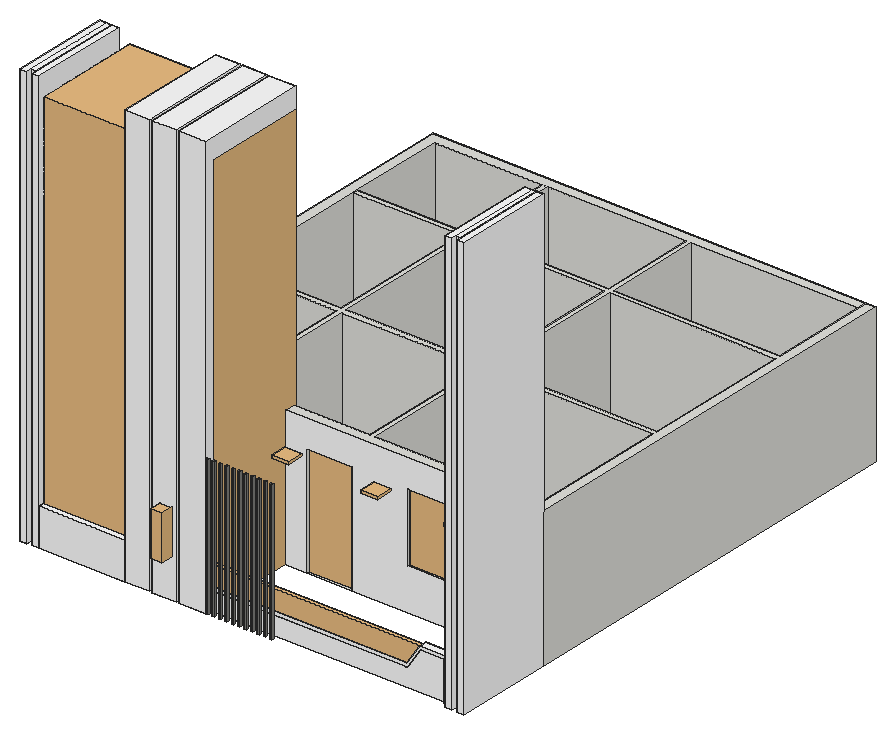
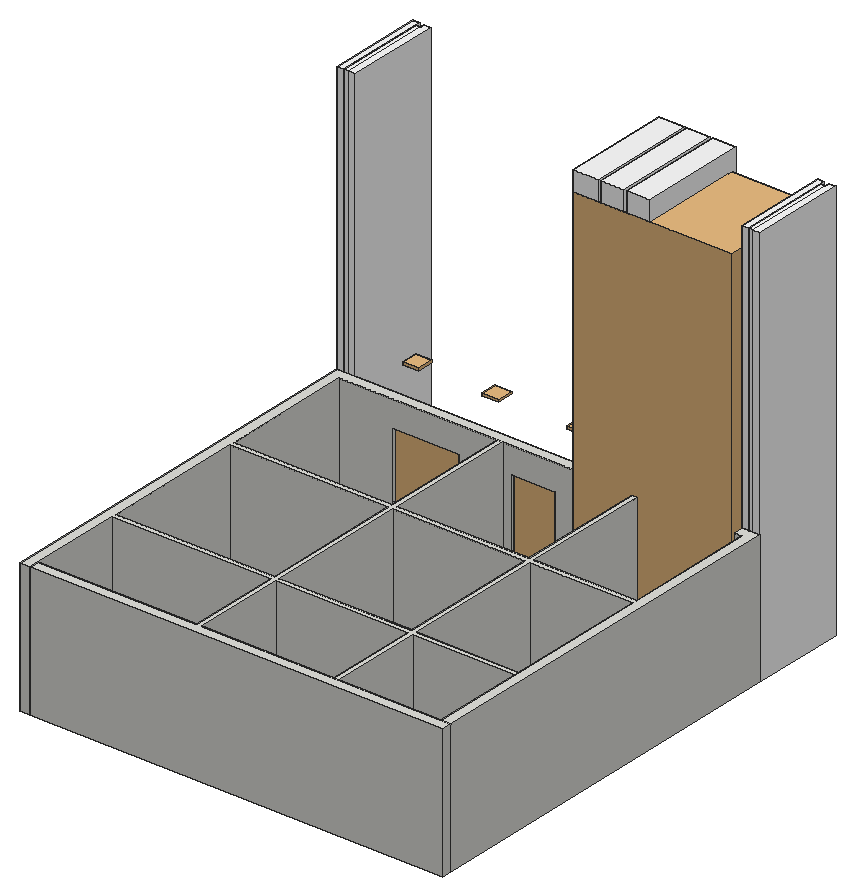
# SketchUp Ruby script. Lengths in inches.
U = 1.inch
M = Sketchup.active_model
def pt(a) = Geom::Point3d.new(a.map { |v| v * U })
def face(e, loops, mat)
  f = e.add_face(loops[0].map { |a| pt(a) })
  loops[1..].each { |l| e.add_face(l.map { |a| pt(a) }).erase! }
  f.material = f.back_material = mat if mat
  f
end
# faces: each face lists its corners as indices into pts; further lists are holes
def faces(e, pts, list, mat = nil) = list.each { |f| face(e, (f[0].is_a?(Array) ? f : [f]).map { |l| l.map { |i| pts[i] } }, mat) }
# xy, xz, yz: faces in a plane at the given z, y or x. An outline is a flat list of corners, or four numbers for a rectangle; further outlines are holes
def ring(l) = l.size == 4 ? [[l[0], l[1]], [l[2], l[1]], [l[2], l[3]], [l[0], l[3]]] : l.each_slice(2).to_a
def flat(e, list, mat, &to3) = list.each { |f| face(e, (f[0].is_a?(Array) ? f : [f]).map { |l| ring(l).map { |u, v| to3.(u, v) } }, mat) }
def xy(e, z, list, mat = nil) = flat(e, list, mat) { |x, y| [x, y, z] }
def xz(e, y, list, mat = nil) = flat(e, list, mat) { |x, z| [x, y, z] }
def yz(e, x, list, mat = nil) = flat(e, list, mat) { |y, z| [x, y, z] }
def lines(e, pts, list) = list.each { |a, b| e.add_line(pt(pts[a]), pt(pts[b])) }
# prism: a flat outline (further loops are holes) pulled along v
def prism(e, loops, v, mat = nil)
  f = face(e, loops, mat); d = Geom::Vector3d.new(v.map { |x| x * U })
  f.pushpull(f.normal.samedirection?(d) ? d.length : -d.length)
end
def box(e, o, s, mat = nil) = prism(e, [[o, [o[0] + s[0], o[1], o[2]], [o[0] + s[0], o[1] + s[1], o[2]], [o[0], o[1] + s[1], o[2]]]], [0, 0, s[2]], mat)
def at(x, y, z, deg = 0) = Geom::Transformation.translation(pt([x, y, z])) * Geom::Transformation.rotation(ORIGIN, Z_AXIS, deg.degrees)
def axes(o, x, y, z) = Geom::Transformation.new([*x, 0, *y, 0, *z, 0, *pt(o).to_a, 1])
def part(name) = M.definitions.add(name)
# library, detail: a bought-in or finely detailed component or shape, given as its bounding box
def library(name, o, s) = part(name).tap { |d| box(d.entities, o, s) }
def detail(e, o, s) = box(e.add_group.entities, o, s)
def put(e, d, t, mat = nil) = e.add_instance(d, t).tap { |i| i.material = mat if mat }
def group(e, t, mat = nil) = e.add_group.tap { |g| g.transformation = t; g.material = mat if mat }.entities
root = M.entities
M.materials.add("Ecorel - epc61025 33.57cm").color = [255, 255, 255]
M.materials.add("Foil Dark Green Matte 0.01cm").color = [255, 255, 255]
M.materials.add("Iron Rough 15cm").color = [129, 129, 125]
M.materials.add("Kamosho - kamn7918 33.43cm").color = [255, 255, 255]
M.materials.add("Leather Brown Alcantara 003 9.18cm").color = [255, 255, 255]
M.materials.add("Pp-1846-msg 17.72cm").color = [255, 255, 255]
c1 = library("Window Crafter Sliding",[0,-0.55,0],[60,4.49,60])
c2 = library("Door 243 065",[-19.36,-2.49,0],[38.72,4.98,81.96])
c3 = library("Group\#13",[0,4.3125,0],[144.25,93,348])
c4 = part("Group\#15")
prism(c4.entities,[[[-3.75,7.71,0],[-3.75,0,0],[-3.75,0,365.875],[-3.75,97.71,365.875],[-3.75,97.71,348],[-3.75,7.71,348]]],[21.11,0,0])
c5 = part("Vertical post")
box(c5.entities,[0,0.5,0],[2,1.5,120],"Iron Rough 15cm")
c6 = part("Stair tread")
box(c6.entities,[0,0,0],[12,36,7])
c7 = part("Stair tread \#1")
box(c7.entities,[0,0,0],[19.0625,36,7])
c8 = part("Stair landing")
box(c8.entities,[-12.25,0,0],[24.25,74,7])
c9 = library("Group\#40",[0,0,0],[184.84,3.15,25.98])
c10 = library("Group\#44",[0,0,0],[10.21,10.4,38.37])
c11 = library("Tlon Light 650 Ceiling 152 007",[-12.8,-12.8,-3.78],[25.6,25.6,3.58])
xy(root,132,[[689.2,386.76,763.65,394.47],[1035.98,391.51,1035.98,391.76,833.45,391.76,833.45,398.76,1040.7,398.76,1040.7,391.51]])
xy(root,148.48,[[833.45,391.51,1004.61,391.76]])
xy(root,151,[[833.45,391.51,1003.26,398.76]],"Foil Dark Green Matte 0.01cm")
xy(root,164.8125,[[689.2,386.76,763.65,394.47]],"Leather Brown Alcantara 003 9.18cm")
xy(root,165.48,[[1015.86,391.51,1035.98,391.76]])
xy(root,168,[[1014.5,391.51,1040.7,398.76]],"Foil Dark Green Matte 0.01cm")
xz(root,386.76,[[689.2,132,763.65,164.8125]],"Leather Brown Alcantara 003 9.18cm")
xz(root,391.51,[[1035.98,132,1040.7,132,1040.7,168,1014.5,168,1003.26,151,833.45,151,833.45,148.48,1004.61,148.48,1015.86,165.48,1035.98,165.48]],"Foil Dark Green Matte 0.01cm")
xz(root,391.76,[[833.45,132,1035.98,132,1035.98,165.48,1015.86,165.48,1004.61,148.48,833.45,148.48]],"Kamosho - kamn7918 33.43cm")
xz(root,394.47,[[689.2,132,763.65,164.8125]])
xz(root,398.76,[[833.45,132,833.45,151,1003.26,151,1014.5,168,1040.7,168,1040.7,132]])
yz(root,689.2,[[386.76,132,394.47,164.8125]])
yz(root,763.65,[[386.76,132,394.47,164.8125]])
yz(root,833.45,[[391.76,132,391.76,148.48,391.51,148.48,391.51,151,398.76,151,398.76,132]])
yz(root,1035.98,[[391.51,132,391.76,165.48]])
yz(root,1040.7,[[391.51,132,398.76,168]])
p = [[1004.61,391.76,148.48],[1015.86,391.76,165.48],[1015.86,391.51,165.48],[1004.61,391.51,148.48],[1003.26,398.76,151],[1003.26,391.51,151],
  [1014.5,391.51,168],[1014.5,398.76,168]]
faces(root,p,[[0,1,2,3]])
faces(root,p,[[4,5,6,7]],"Foil Dark Green Matte 0.01cm")
g1 = group(root,at(672.95,472.76,132))
put(g1,c1,at(266.5625,2.73,36))
put(g1,c2,axes([198.48,4.93,0],[1,0,0],[0,1,0],[0,0,1.17128]))
g2 = group(g1,at(0,0,0))
xy(g2,0,[[179.1875,0,218.1875,9],[9,9,102,129],[106.5,9,226.5,129],[231,9,375,129],[9,133.5,102,262.5],
  [106.5,133.5,226.5,262.5],[231,133.5,375,262.5],[9,267,102,351],[106.5,267,226.5,351],[231,267,375,351]])
xy(g2,36,[[266.5625,0,326.5625,9]])
xy(g2,96,[[179.1875,0,218.1875,9],[266.5625,0,326.5625,9]])
xy(g2,120,[[[0,0,384,0,384,360,375,360,375,267,231,267,231,351,375,351,375,360,0,360,0,351,226.5,351,226.5,267,106.5,267,106.5,351,102,351,102,267,9,267,9,262.5,102,262.5,102,133.5,9,133.5,9,351,0,351],[106.5,9,106.5,129,226.5,129,226.5,9,231,9,231,129,375,129,375,9],[231,133.5,375,262.5],[106.5,133.5,226.5,262.5],[9,9,102,129]]])
xz(g2,0,[[[0,0,179.1875,0,179.1875,96,218.1875,96,218.1875,0,384,0,384,120,0,120],[266.5625,36,326.5625,96]]],"Pp-1846-msg 17.72cm")
xz(g2,9,[[9,0,102,120],[106.5,0,106.5,120,226.5,120,226.5,0,218.1875,0,218.1875,96,179.1875,96,179.1875,0],[226.5,0,231,120],[[231,0,375,120],[266.5625,36,326.5625,96]]])
xz(g2,129,[[9,0,102,120],[106.5,0,226.5,120],[231,0,375,120]])
xz(g2,133.5,[[9,0,102,120],[106.5,0,226.5,120],[231,0,375,120]])
xz(g2,262.5,[[9,0,102,120],[106.5,0,226.5,120],[231,0,375,120]])
xz(g2,267,[[9,0,102,120],[106.5,0,226.5,120],[231,0,375,120]])
xz(g2,351,[[0,0,9,120],[9,0,102,120],[102,0,106.5,120],[106.5,0,226.5,120],[231,0,375,120]])
xz(g2,360,[[0,0,375,120],[375,0,384,120]])
yz(g2,0,[[0,0,351,120],[351,0,360,120]])
yz(g2,9,[[9,0,129,120],[133.5,0,262.5,120],[262.5,0,267,120],[267,0,351,120]])
yz(g2,102,[[9,0,129,120],[133.5,0,262.5,120],[267,0,351,120]])
yz(g2,106.5,[[9,0,129,120],[133.5,0,262.5,120],[267,0,351,120]])
yz(g2,179.1875,[[0,0,9,96]])
yz(g2,218.1875,[[0,0,9,96]])
yz(g2,226.5,[[9,0,129,120],[133.5,0,262.5,120],[267,0,351,120]])
yz(g2,231,[[9,0,129,120],[133.5,0,262.5,120],[267,0,351,120]])
yz(g2,266.5625,[[0,36,9,96]])
yz(g2,326.5625,[[0,36,9,96]])
yz(g2,375,[[9,0,129,120],[133.5,0,262.5,120],[267,0,351,120],[351,0,360,120]])
yz(g2,384,[[0,0,360,120]])
g3 = group(root,at(1040.7,398.76,132),"Ecorel - epc61025 33.57cm")
xy(g3,0,[[0,-12,6,74],[6,-7.96,10.25,74]])
xy(g3,365.875,[[0,-12,6,74],[6,-7.96,10.25,74]])
xz(g3,-12,[[0,0,6,365.875]])
xz(g3,-7.96,[[6,0,10.25,365.875]],"Foil Dark Green Matte 0.01cm")
xz(g3,74,[[0,0,6,365.875],[6,0,10.25,365.875]])
yz(g3,0,[[-12,0,74,365.875]])
yz(g3,6,[[-12,0,-7.96,365.875]])
yz(g3,10.25,[[-7.96,0,74,365.875]])
g4 = group(g3,at(10.25,0,0))
box(g4,[0,-12,0],[6,86,365.875])
g5 = group(root,at(672.95,398.76,132),"Leather Brown Alcantara 003 9.18cm")
xy(g5,0,[[0,-12,6,74],[6,-7.96,10.25,74]])
xy(g5,365.875,[[0,-12,6,74],[6,-7.96,10.25,74]])
xz(g5,-12,[[0,0,6,365.875]])
xz(g5,-7.96,[[6,0,10.25,365.875]],"Foil Dark Green Matte 0.01cm")
xz(g5,74,[[0,0,6,365.875],[6,0,10.25,365.875]])
yz(g5,0,[[-12,0,74,365.875]])
yz(g5,6,[[-12,0,-7.96,365.875]])
yz(g5,10.25,[[-7.96,0,74,365.875]])
g6 = group(g5,at(10.25,0,0))
box(g6,[0,-12,0],[6,86,365.875])
put(root,c3,at(689.2,387.16,132),"Ecorel - epc61025 33.57cm")
g7 = group(root,at(813.71,386.76,132),"Leather Brown Alcantara 003 9.18cm")
prism(g7,[[[-3.75,7.71,0],[-3.75,0,0],[-3.75,0,365.875],[-3.75,97.71,365.875],[-3.75,97.71,348],[-3.75,7.71,348]]],[23.49,0,0])
put(root,c4,at(767.4,386.76,132),"Leather Brown Alcantara 003 9.18cm")
g8 = group(root,at(833.45,386.76,132))
put(g8,c5,at(0,-0.5,0))
g9 = group(g8,at(5.55,0,0))
put(g9,c5,at(11.09,-0.5,0))
put(g9,c5,at(22.1875,-0.5,0))
put(g9,c5,at(27.73,-0.5,0))
put(g9,c5,at(16.64,-0.5,0))
put(g9,c5,at(49.92,-0.5,0))
put(g9,c5,at(44.37,-0.5,0))
put(g9,c5,at(0,-0.5,0))
put(g9,c5,at(33.28,-0.5,0))
put(g9,c5,at(5.55,-0.5,0))
put(g9,c5,at(38.83,-0.5,0))
put(root,c4,at(790.9,386.76,132),"Leather Brown Alcantara 003 9.18cm")
g10 = group(root,at(677.45,398.76,132))
put(g10,c6,at(36,38,77))
put(g10,c6,at(132,0,7))
put(g10,c6,at(108,0,21))
put(g10,c6,at(120,0,14))
put(g10,c6,at(144,0,0))
put(g10,c6,at(60,38,91))
put(g10,c6,at(84,38,105))
put(g10,c6,at(96,38,112))
put(g10,c6,at(48,38,84))
put(g10,c7,at(108,38,119))
put(g10,c6,at(72,38,98))
put(g10,c6,at(48,0,56))
put(g10,c6,at(60,0,49))
put(g10,c8,at(24,0,70))
put(g10,c6,at(36,0,63))
put(g10,c6,at(84,0,35))
put(g10,c6,at(96,0,28))
put(g10,c6,at(72,0,42))
put(root,c9,axes([831.48,392.89,151],[0.99016,0,0],[0,1,0],[0,0,0.65424]))
put(root,c10,at(793.58,376.76,165.39))
put(root,c11,axes([871.45,426.96,251.11],[0.58,0,0],[0,0.58,0],[0,0,0.58]))
put(root,c11,axes([1020.87,426.96,251.11],[0.58,0,0],[0,0.58,0],[0,0,0.58]))
put(root,c11,axes([948.45,426.96,251.11],[0.58,0,0],[0,0.58,0],[0,0,0.58]))
